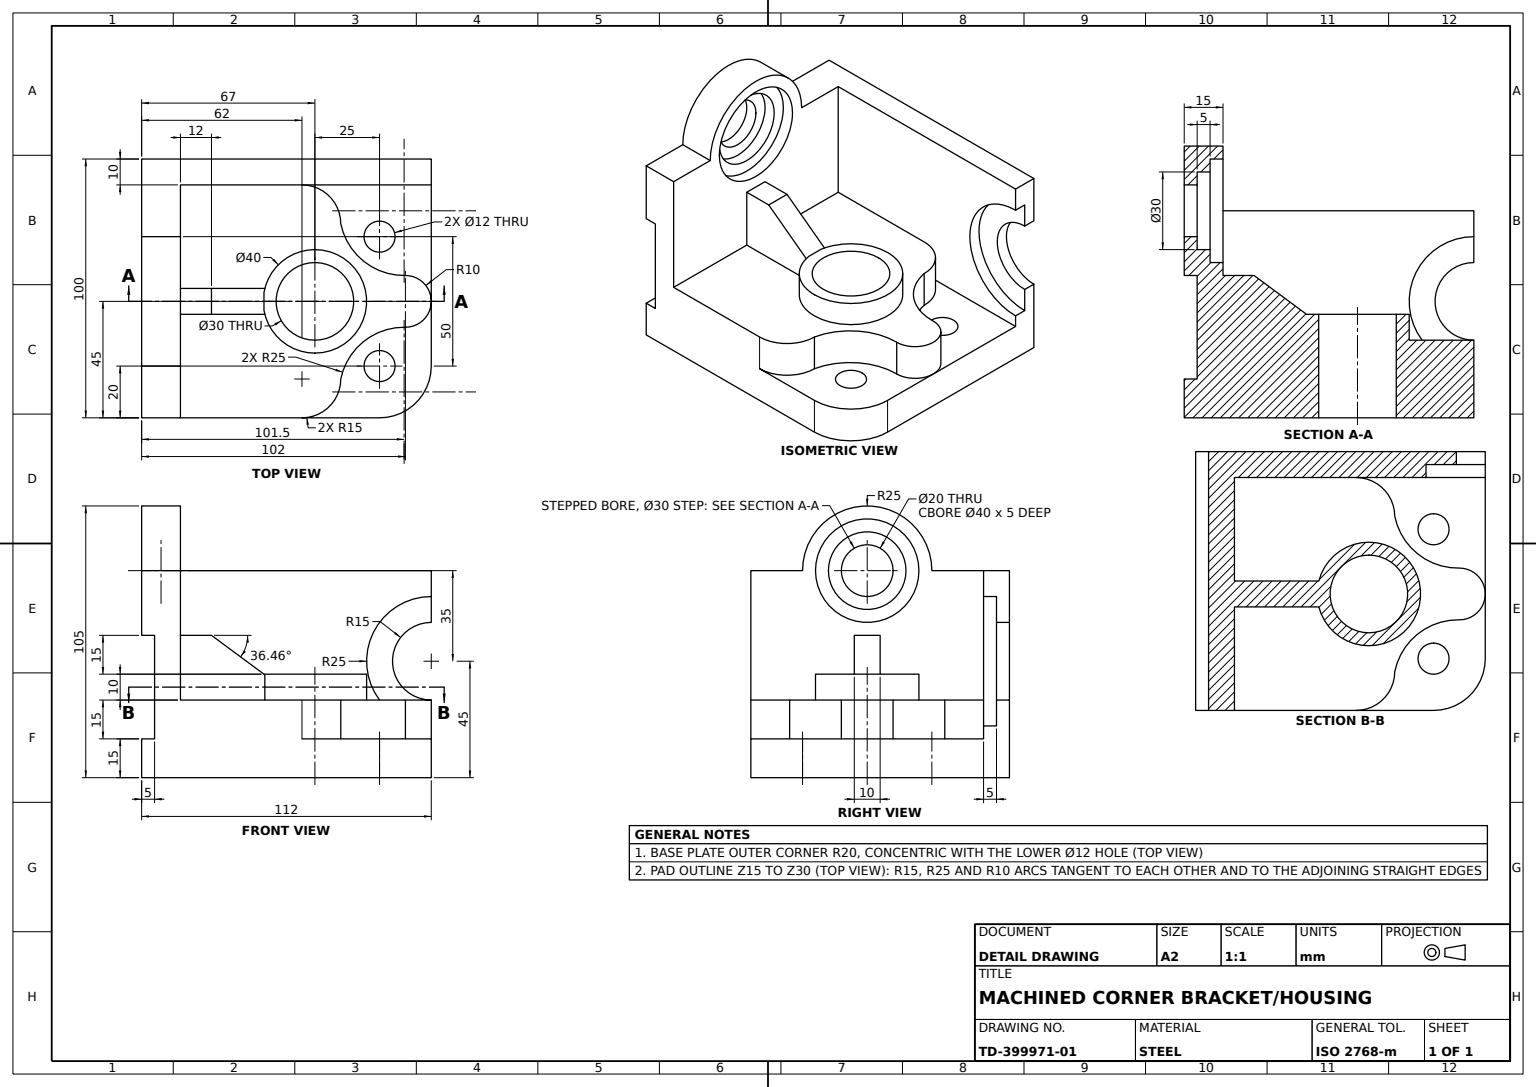
ISO-10303-21;
HEADER;
FILE_DESCRIPTION((''),'2;1');
FILE_NAME('','',(''),(''),'','','');
FILE_SCHEMA(('AUTOMOTIVE_DESIGN'));
ENDSEC;
DATA;
#1=APPLICATION_CONTEXT('');
#2=PRODUCT_CONTEXT('',#1,'mechanical');
#3=PRODUCT('','','',(#2));
#4=PRODUCT_DEFINITION_FORMATION('','',#3);
#5=PRODUCT_DEFINITION_CONTEXT('',#1,'design');
#6=PRODUCT_DEFINITION('','',#4,#5);
#7=PRODUCT_DEFINITION_SHAPE('','',#6);
#8=(LENGTH_UNIT()NAMED_UNIT(*)SI_UNIT(.MILLI.,.METRE.));
#9=(NAMED_UNIT(*)PLANE_ANGLE_UNIT()SI_UNIT($,.RADIAN.));
#10=(NAMED_UNIT(*)SI_UNIT($,.STERADIAN.)SOLID_ANGLE_UNIT());
#11=UNCERTAINTY_MEASURE_WITH_UNIT(LENGTH_MEASURE(1.E-05),#8,'distance_accuracy_value','');
#12=(GEOMETRIC_REPRESENTATION_CONTEXT(3)GLOBAL_UNCERTAINTY_ASSIGNED_CONTEXT((#11))GLOBAL_UNIT_ASSIGNED_CONTEXT((#8,#9,#10))REPRESENTATION_CONTEXT('',''));
#13=CARTESIAN_POINT('',(0.,40.,15.));
#14=VERTEX_POINT('',#13);
#15=CARTESIAN_POINT('',(0.,40.,-15.));
#16=VERTEX_POINT('',#15);
#17=CARTESIAN_POINT('',(0.,40.,0.));
#18=DIRECTION('',(0.,1.,0.));
#19=DIRECTION('',(0.,0.,1.));
#20=AXIS2_PLACEMENT_3D('',#17,#18,#19);
#21=CIRCLE('',#20,15.);
#22=EDGE_CURVE('',#14,#16,#21,.T.);
#23=ORIENTED_EDGE('',*,*,#22,.T.);
#24=CARTESIAN_POINT('',(0.,0.,-15.));
#25=VERTEX_POINT('',#24);
#26=DIRECTION('',(0.,-1.,0.));
#27=VECTOR('',#26,1000.);
#28=LINE('',#15,#27);
#29=EDGE_CURVE('',#16,#25,#28,.T.);
#30=ORIENTED_EDGE('',*,*,#29,.T.);
#31=CARTESIAN_POINT('',(0.,0.,15.));
#32=VERTEX_POINT('',#31);
#33=CARTESIAN_POINT('',(0.,0.,0.));
#34=AXIS2_PLACEMENT_3D('',#33,#18,#19);
#35=CIRCLE('',#34,15.);
#36=EDGE_CURVE('',#32,#25,#35,.T.);
#37=ORIENTED_EDGE('',*,*,#36,.F.);
#38=LINE('',#13,#27);
#39=EDGE_CURVE('',#14,#32,#38,.T.);
#40=ORIENTED_EDGE('',*,*,#39,.F.);
#41=EDGE_LOOP('',(#23,#30,#37,#40));
#42=FACE_OUTER_BOUND('',#41,.T.);
#43=DIRECTION('',(0.,0.,-1.));
#44=AXIS2_PLACEMENT_3D('',#17,#26,#43);
#45=CYLINDRICAL_SURFACE('',#44,15.);
#46=ADVANCED_FACE('',(#42),#45,.F.);
#47=CARTESIAN_POINT('',(-62.,80.,15.));
#48=VERTEX_POINT('',#47);
#49=CARTESIAN_POINT('',(-62.,80.,-15.));
#50=VERTEX_POINT('',#49);
#51=CARTESIAN_POINT('',(-62.,80.,0.));
#52=DIRECTION('',(1.,0.,0.));
#53=AXIS2_PLACEMENT_3D('',#51,#52,#43);
#54=CIRCLE('',#53,15.);
#55=EDGE_CURVE('',#48,#50,#54,.T.);
#56=ORIENTED_EDGE('',*,*,#55,.T.);
#57=EDGE_CURVE('',#50,#48,#54,.T.);
#58=ORIENTED_EDGE('',*,*,#57,.T.);
#59=EDGE_LOOP('',(#56,#58));
#60=FACE_OUTER_BOUND('',#59,.T.);
#61=CARTESIAN_POINT('',(-62.,80.,10.));
#62=VERTEX_POINT('',#61);
#63=CARTESIAN_POINT('',(-62.,80.,-10.));
#64=VERTEX_POINT('',#63);
#65=DIRECTION('',(-1.,0.,0.));
#66=AXIS2_PLACEMENT_3D('',#51,#65,#43);
#67=CIRCLE('',#66,10.);
#68=EDGE_CURVE('',#62,#64,#67,.T.);
#69=ORIENTED_EDGE('',*,*,#68,.T.);
#70=EDGE_CURVE('',#64,#62,#67,.T.);
#71=ORIENTED_EDGE('',*,*,#70,.T.);
#72=EDGE_LOOP('',(#69,#71));
#73=FACE_BOUND('',#72,.T.);
#74=PLANE('',#53);
#75=ADVANCED_FACE('',(#60,#73),#74,.T.);
#76=CARTESIAN_POINT('',(-52.,30.,5.));
#77=VERTEX_POINT('',#76);
#78=CARTESIAN_POINT('',(-19.364917,30.,5.));
#79=VERTEX_POINT('',#78);
#80=CARTESIAN_POINT('',(34.495934,30.,5.));
#81=VECTOR('',#52,1000.);
#82=LINE('',#80,#81);
#83=EDGE_CURVE('',#77,#79,#82,.T.);
#84=ORIENTED_EDGE('',*,*,#83,.T.);
#85=CARTESIAN_POINT('',(-19.364917,39.752402,5.));
#86=VERTEX_POINT('',#85);
#87=CARTESIAN_POINT('',(-19.364917,40.,5.));
#88=LINE('',#87,#27);
#89=EDGE_CURVE('',#86,#79,#88,.T.);
#90=ORIENTED_EDGE('',*,*,#89,.F.);
#91=CARTESIAN_POINT('',(-40.,55.,5.));
#92=VERTEX_POINT('',#91);
#93=DIRECTION('',(0.804258471,-0.594279658,0.));
#94=VECTOR('',#93,1000.);
#95=LINE('',#91,#94);
#96=EDGE_CURVE('',#92,#86,#95,.T.);
#97=ORIENTED_EDGE('',*,*,#96,.F.);
#98=CARTESIAN_POINT('',(-52.,55.,5.));
#99=VERTEX_POINT('',#98);
#100=CARTESIAN_POINT('',(-11.,55.,5.));
#101=LINE('',#100,#81);
#102=EDGE_CURVE('',#99,#92,#101,.T.);
#103=ORIENTED_EDGE('',*,*,#102,.F.);
#104=CARTESIAN_POINT('',(-52.,0.,5.));
#105=VECTOR('',#18,1000.);
#106=LINE('',#104,#105);
#107=EDGE_CURVE('',#77,#99,#106,.T.);
#108=ORIENTED_EDGE('',*,*,#107,.F.);
#109=EDGE_LOOP('',(#84,#90,#97,#103,#108));
#110=FACE_OUTER_BOUND('',#109,.T.);
#111=CARTESIAN_POINT('',(-11.,40.,5.));
#112=AXIS2_PLACEMENT_3D('',#111,#19,#52);
#113=PLANE('',#112);
#114=ADVANCED_FACE('',(#110),#113,.T.);
#115=CARTESIAN_POINT('',(-52.,80.,45.));
#116=VERTEX_POINT('',#115);
#117=CARTESIAN_POINT('',(-67.,80.,45.));
#118=VERTEX_POINT('',#117);
#119=CARTESIAN_POINT('',(0.,80.,45.));
#120=VECTOR('',#65,1000.);
#121=LINE('',#119,#120);
#122=EDGE_CURVE('',#116,#118,#121,.T.);
#123=ORIENTED_EDGE('',*,*,#122,.F.);
#124=CARTESIAN_POINT('',(-52.,80.,25.));
#125=VERTEX_POINT('',#124);
#126=CARTESIAN_POINT('',(-52.,80.,-45.));
#127=VECTOR('',#19,1000.);
#128=LINE('',#126,#127);
#129=EDGE_CURVE('',#125,#116,#128,.T.);
#130=ORIENTED_EDGE('',*,*,#129,.F.);
#131=CARTESIAN_POINT('',(-67.,80.,25.));
#132=VERTEX_POINT('',#131);
#133=LINE('',#131,#81);
#134=EDGE_CURVE('',#132,#125,#133,.T.);
#135=ORIENTED_EDGE('',*,*,#134,.F.);
#136=CARTESIAN_POINT('',(-67.,80.,-45.));
#137=LINE('',#136,#127);
#138=EDGE_CURVE('',#132,#118,#137,.T.);
#139=ORIENTED_EDGE('',*,*,#138,.T.);
#140=EDGE_LOOP('',(#123,#130,#135,#139));
#141=FACE_OUTER_BOUND('',#140,.T.);
#142=CARTESIAN_POINT('',(0.,80.,-45.));
#143=AXIS2_PLACEMENT_3D('',#142,#18,#19);
#144=PLANE('',#143);
#145=ADVANCED_FACE('',(#141),#144,.T.);
#146=CARTESIAN_POINT('',(-67.,0.,-55.));
#147=VERTEX_POINT('',#146);
#148=CARTESIAN_POINT('',(45.,0.,-55.));
#149=VERTEX_POINT('',#148);
#150=LINE('',#146,#81);
#151=EDGE_CURVE('',#147,#149,#150,.T.);
#152=ORIENTED_EDGE('',*,*,#151,.F.);
#153=CARTESIAN_POINT('',(-67.,15.,-55.));
#154=VERTEX_POINT('',#153);
#155=CARTESIAN_POINT('',(-67.,-112.445542,-55.));
#156=LINE('',#155,#105);
#157=EDGE_CURVE('',#147,#154,#156,.T.);
#158=ORIENTED_EDGE('',*,*,#157,.T.);
#159=CARTESIAN_POINT('',(-62.,15.,-55.));
#160=VERTEX_POINT('',#159);
#161=LINE('',#153,#120);
#162=EDGE_CURVE('',#160,#154,#161,.T.);
#163=ORIENTED_EDGE('',*,*,#162,.F.);
#164=CARTESIAN_POINT('',(-62.,55.,-55.));
#165=VERTEX_POINT('',#164);
#166=CARTESIAN_POINT('',(-62.,-112.445542,-55.));
#167=LINE('',#166,#27);
#168=EDGE_CURVE('',#165,#160,#167,.T.);
#169=ORIENTED_EDGE('',*,*,#168,.F.);
#170=CARTESIAN_POINT('',(-67.,55.,-55.));
#171=VERTEX_POINT('',#170);
#172=LINE('',#170,#81);
#173=EDGE_CURVE('',#171,#165,#172,.T.);
#174=ORIENTED_EDGE('',*,*,#173,.F.);
#175=CARTESIAN_POINT('',(-67.,80.,-55.));
#176=VERTEX_POINT('',#175);
#177=EDGE_CURVE('',#171,#176,#156,.T.);
#178=ORIENTED_EDGE('',*,*,#177,.T.);
#179=CARTESIAN_POINT('',(45.,80.,-55.));
#180=VERTEX_POINT('',#179);
#181=LINE('',#175,#120);
#182=EDGE_CURVE('',#180,#176,#181,.T.);
#183=ORIENTED_EDGE('',*,*,#182,.F.);
#184=CARTESIAN_POINT('',(45.,60.,-55.));
#185=VERTEX_POINT('',#184);
#186=CARTESIAN_POINT('',(45.,-112.445542,-55.));
#187=LINE('',#186,#105);
#188=EDGE_CURVE('',#185,#180,#187,.T.);
#189=ORIENTED_EDGE('',*,*,#188,.F.);
#190=CARTESIAN_POINT('',(45.,30.,-55.));
#191=VERTEX_POINT('',#190);
#192=CARTESIAN_POINT('',(45.,45.,-55.));
#193=AXIS2_PLACEMENT_3D('',#192,#19,#52);
#194=CIRCLE('',#193,15.);
#195=EDGE_CURVE('',#185,#191,#194,.T.);
#196=ORIENTED_EDGE('',*,*,#195,.T.);
#197=EDGE_CURVE('',#149,#191,#187,.T.);
#198=ORIENTED_EDGE('',*,*,#197,.F.);
#199=EDGE_LOOP('',(#152,#158,#163,#169,#174,#178,#183,#189,#196,#198));
#200=FACE_OUTER_BOUND('',#199,.T.);
#201=AXIS2_PLACEMENT_3D('',#155,#43,#65);
#202=PLANE('',#201);
#203=ADVANCED_FACE('',(#200),#202,.T.);
#204=CARTESIAN_POINT('',(-5.,30.,-45.));
#205=VERTEX_POINT('',#204);
#206=CARTESIAN_POINT('',(-5.,15.,-45.));
#207=VERTEX_POINT('',#206);
#208=LINE('',#204,#27);
#209=EDGE_CURVE('',#205,#207,#208,.T.);
#210=ORIENTED_EDGE('',*,*,#209,.F.);
#211=CARTESIAN_POINT('',(10.,30.,-30.));
#212=VERTEX_POINT('',#211);
#213=CARTESIAN_POINT('',(-5.,30.,-30.));
#214=AXIS2_PLACEMENT_3D('',#213,#18,#19);
#215=CIRCLE('',#214,15.);
#216=EDGE_CURVE('',#212,#205,#215,.T.);
#217=ORIENTED_EDGE('',*,*,#216,.F.);
#218=CARTESIAN_POINT('',(10.,15.,-30.));
#219=VERTEX_POINT('',#218);
#220=LINE('',#211,#27);
#221=EDGE_CURVE('',#212,#219,#220,.T.);
#222=ORIENTED_EDGE('',*,*,#221,.T.);
#223=CARTESIAN_POINT('',(-5.,15.,-30.));
#224=AXIS2_PLACEMENT_3D('',#223,#18,#19);
#225=CIRCLE('',#224,15.);
#226=EDGE_CURVE('',#219,#207,#225,.T.);
#227=ORIENTED_EDGE('',*,*,#226,.T.);
#228=EDGE_LOOP('',(#210,#217,#222,#227));
#229=FACE_OUTER_BOUND('',#228,.T.);
#230=AXIS2_PLACEMENT_3D('',#213,#26,#43);
#231=CYLINDRICAL_SURFACE('',#230,15.);
#232=ADVANCED_FACE('',(#229),#231,.T.);
#233=CARTESIAN_POINT('',(45.,15.,-45.));
#234=VERTEX_POINT('',#233);
#235=CARTESIAN_POINT('',(-45.,15.,-45.));
#236=LINE('',#235,#120);
#237=EDGE_CURVE('',#234,#207,#236,.T.);
#238=ORIENTED_EDGE('',*,*,#237,.T.);
#239=ORIENTED_EDGE('',*,*,#226,.F.);
#240=CARTESIAN_POINT('',(35.,15.,-10.));
#241=VERTEX_POINT('',#240);
#242=CARTESIAN_POINT('',(34.495934,15.,-34.994918));
#243=AXIS2_PLACEMENT_3D('',#242,#26,#19);
#244=CIRCLE('',#243,25.);
#245=EDGE_CURVE('',#241,#219,#244,.T.);
#246=ORIENTED_EDGE('',*,*,#245,.F.);
#247=CARTESIAN_POINT('',(45.,15.,0.));
#248=VERTEX_POINT('',#247);
#249=CARTESIAN_POINT('',(35.,15.,0.));
#250=AXIS2_PLACEMENT_3D('',#249,#18,#19);
#251=CIRCLE('',#250,10.);
#252=EDGE_CURVE('',#248,#241,#251,.T.);
#253=ORIENTED_EDGE('',*,*,#252,.F.);
#254=VECTOR('',#43,1000.);
#255=LINE('',#233,#254);
#256=EDGE_CURVE('',#248,#234,#255,.T.);
#257=ORIENTED_EDGE('',*,*,#256,.T.);
#258=EDGE_LOOP('',(#238,#239,#246,#253,#257));
#259=FACE_OUTER_BOUND('',#258,.T.);
#260=CARTESIAN_POINT('',(25.,15.,-31.));
#261=VERTEX_POINT('',#260);
#262=CARTESIAN_POINT('',(25.,15.,-19.));
#263=VERTEX_POINT('',#262);
#264=CARTESIAN_POINT('',(25.,15.,-25.));
#265=AXIS2_PLACEMENT_3D('',#264,#18,#19);
#266=CIRCLE('',#265,6.);
#267=EDGE_CURVE('',#261,#263,#266,.T.);
#268=ORIENTED_EDGE('',*,*,#267,.F.);
#269=EDGE_CURVE('',#263,#261,#266,.T.);
#270=ORIENTED_EDGE('',*,*,#269,.F.);
#271=EDGE_LOOP('',(#268,#270));
#272=FACE_BOUND('',#271,.T.);
#273=CARTESIAN_POINT('',(25.,15.,25.));
#274=AXIS2_PLACEMENT_3D('',#273,#18,#19);
#275=PLANE('',#274);
#276=ADVANCED_FACE('',(#259,#272),#275,.T.);
#277=CARTESIAN_POINT('',(45.,60.,-50.));
#278=VERTEX_POINT('',#277);
#279=CARTESIAN_POINT('',(45.,70.,-50.));
#280=VERTEX_POINT('',#279);
#281=CARTESIAN_POINT('',(45.,15.,-50.));
#282=LINE('',#281,#105);
#283=EDGE_CURVE('',#278,#280,#282,.T.);
#284=ORIENTED_EDGE('',*,*,#283,.T.);
#285=CARTESIAN_POINT('',(45.,20.,-50.));
#286=VERTEX_POINT('',#285);
#287=CARTESIAN_POINT('',(45.,45.,-50.));
#288=AXIS2_PLACEMENT_3D('',#287,#19,#52);
#289=CIRCLE('',#288,25.);
#290=EDGE_CURVE('',#280,#286,#289,.T.);
#291=ORIENTED_EDGE('',*,*,#290,.T.);
#292=CARTESIAN_POINT('',(45.,30.,-50.));
#293=VERTEX_POINT('',#292);
#294=EDGE_CURVE('',#286,#293,#282,.T.);
#295=ORIENTED_EDGE('',*,*,#294,.T.);
#296=CIRCLE('',#288,15.);
#297=EDGE_CURVE('',#278,#293,#296,.T.);
#298=ORIENTED_EDGE('',*,*,#297,.F.);
#299=EDGE_LOOP('',(#284,#291,#295,#298));
#300=FACE_OUTER_BOUND('',#299,.T.);
#301=PLANE('',#288);
#302=ADVANCED_FACE('',(#300),#301,.T.);
#303=CARTESIAN_POINT('',(-52.,30.,45.));
#304=VERTEX_POINT('',#303);
#305=CARTESIAN_POINT('',(-52.,0.,45.));
#306=LINE('',#305,#27);
#307=EDGE_CURVE('',#116,#304,#306,.T.);
#308=ORIENTED_EDGE('',*,*,#307,.T.);
#309=CARTESIAN_POINT('',(-52.,30.,-45.));
#310=LINE('',#309,#127);
#311=EDGE_CURVE('',#77,#304,#310,.T.);
#312=ORIENTED_EDGE('',*,*,#311,.F.);
#313=ORIENTED_EDGE('',*,*,#107,.T.);
#314=CARTESIAN_POINT('',(-52.,55.,-5.));
#315=VERTEX_POINT('',#314);
#316=CARTESIAN_POINT('',(-52.,55.,-45.));
#317=LINE('',#316,#254);
#318=EDGE_CURVE('',#99,#315,#317,.T.);
#319=ORIENTED_EDGE('',*,*,#318,.T.);
#320=CARTESIAN_POINT('',(-52.,30.,-5.));
#321=VERTEX_POINT('',#320);
#322=CARTESIAN_POINT('',(-52.,0.,-5.));
#323=LINE('',#322,#105);
#324=EDGE_CURVE('',#321,#315,#323,.T.);
#325=ORIENTED_EDGE('',*,*,#324,.F.);
#326=VERTEX_POINT('',#309);
#327=EDGE_CURVE('',#326,#321,#310,.T.);
#328=ORIENTED_EDGE('',*,*,#327,.F.);
#329=VERTEX_POINT('',#126);
#330=CARTESIAN_POINT('',(-52.,0.,-45.));
#331=LINE('',#330,#27);
#332=EDGE_CURVE('',#329,#326,#331,.T.);
#333=ORIENTED_EDGE('',*,*,#332,.F.);
#334=CARTESIAN_POINT('',(-52.,80.,-25.));
#335=VERTEX_POINT('',#334);
#336=EDGE_CURVE('',#329,#335,#128,.T.);
#337=ORIENTED_EDGE('',*,*,#336,.T.);
#338=CARTESIAN_POINT('',(-52.,80.,0.));
#339=AXIS2_PLACEMENT_3D('',#338,#52,#43);
#340=CIRCLE('',#339,25.);
#341=EDGE_CURVE('',#335,#125,#340,.T.);
#342=ORIENTED_EDGE('',*,*,#341,.T.);
#343=ORIENTED_EDGE('',*,*,#129,.T.);
#344=EDGE_LOOP('',(#308,#312,#313,#319,#325,#328,#333,#337,#342,#343));
#345=FACE_OUTER_BOUND('',#344,.T.);
#346=CARTESIAN_POINT('',(-52.,80.,20.));
#347=VERTEX_POINT('',#346);
#348=CARTESIAN_POINT('',(-52.,80.,-20.));
#349=VERTEX_POINT('',#348);
#350=CIRCLE('',#339,20.);
#351=EDGE_CURVE('',#347,#349,#350,.T.);
#352=ORIENTED_EDGE('',*,*,#351,.F.);
#353=EDGE_CURVE('',#349,#347,#350,.T.);
#354=ORIENTED_EDGE('',*,*,#353,.F.);
#355=EDGE_LOOP('',(#352,#354));
#356=FACE_BOUND('',#355,.T.);
#357=AXIS2_PLACEMENT_3D('',#330,#65,#19);
#358=PLANE('',#357);
#359=ADVANCED_FACE('',(#345,#356),#358,.F.);
#360=CARTESIAN_POINT('',(25.,15.,19.));
#361=VERTEX_POINT('',#360);
#362=CARTESIAN_POINT('',(25.,15.,31.));
#363=VERTEX_POINT('',#362);
#364=CIRCLE('',#274,6.);
#365=EDGE_CURVE('',#361,#363,#364,.T.);
#366=ORIENTED_EDGE('',*,*,#365,.F.);
#367=EDGE_CURVE('',#363,#361,#364,.T.);
#368=ORIENTED_EDGE('',*,*,#367,.F.);
#369=EDGE_LOOP('',(#366,#368));
#370=FACE_BOUND('',#369,.T.);
#371=CARTESIAN_POINT('',(45.,15.,25.));
#372=VERTEX_POINT('',#371);
#373=EDGE_CURVE('',#372,#248,#255,.T.);
#374=ORIENTED_EDGE('',*,*,#373,.T.);
#375=CARTESIAN_POINT('',(35.,15.,10.));
#376=VERTEX_POINT('',#375);
#377=EDGE_CURVE('',#376,#248,#251,.T.);
#378=ORIENTED_EDGE('',*,*,#377,.F.);
#379=CARTESIAN_POINT('',(34.495934,15.,9.994918));
#380=VERTEX_POINT('',#379);
#381=CARTESIAN_POINT('',(34.495934,15.,34.994918));
#382=AXIS2_PLACEMENT_3D('',#381,#26,#43);
#383=CIRCLE('',#382,25.);
#384=EDGE_CURVE('',#380,#376,#383,.T.);
#385=ORIENTED_EDGE('',*,*,#384,.F.);
#386=CARTESIAN_POINT('',(10.,15.,30.));
#387=VERTEX_POINT('',#386);
#388=EDGE_CURVE('',#387,#380,#383,.T.);
#389=ORIENTED_EDGE('',*,*,#388,.F.);
#390=CARTESIAN_POINT('',(-5.,15.,45.));
#391=VERTEX_POINT('',#390);
#392=CARTESIAN_POINT('',(-5.,15.,30.));
#393=AXIS2_PLACEMENT_3D('',#392,#18,#19);
#394=CIRCLE('',#393,15.);
#395=EDGE_CURVE('',#391,#387,#394,.T.);
#396=ORIENTED_EDGE('',*,*,#395,.F.);
#397=CARTESIAN_POINT('',(25.,15.,45.));
#398=VERTEX_POINT('',#397);
#399=CARTESIAN_POINT('',(-45.,15.,45.));
#400=LINE('',#399,#81);
#401=EDGE_CURVE('',#391,#398,#400,.T.);
#402=ORIENTED_EDGE('',*,*,#401,.T.);
#403=CIRCLE('',#274,20.);
#404=EDGE_CURVE('',#398,#372,#403,.T.);
#405=ORIENTED_EDGE('',*,*,#404,.T.);
#406=EDGE_LOOP('',(#374,#378,#385,#389,#396,#402,#405));
#407=FACE_OUTER_BOUND('',#406,.T.);
#408=ADVANCED_FACE('',(#370,#407),#275,.T.);
#409=CARTESIAN_POINT('',(25.,0.,31.));
#410=VERTEX_POINT('',#409);
#411=CARTESIAN_POINT('',(25.,0.,19.));
#412=VERTEX_POINT('',#411);
#413=CARTESIAN_POINT('',(25.,0.,25.));
#414=AXIS2_PLACEMENT_3D('',#413,#18,#19);
#415=CIRCLE('',#414,6.);
#416=EDGE_CURVE('',#410,#412,#415,.T.);
#417=ORIENTED_EDGE('',*,*,#416,.F.);
#418=LINE('',#362,#27);
#419=EDGE_CURVE('',#363,#410,#418,.T.);
#420=ORIENTED_EDGE('',*,*,#419,.F.);
#421=ORIENTED_EDGE('',*,*,#367,.T.);
#422=LINE('',#360,#27);
#423=EDGE_CURVE('',#361,#412,#422,.T.);
#424=ORIENTED_EDGE('',*,*,#423,.T.);
#425=EDGE_LOOP('',(#417,#420,#421,#424));
#426=FACE_OUTER_BOUND('',#425,.T.);
#427=AXIS2_PLACEMENT_3D('',#273,#26,#43);
#428=CYLINDRICAL_SURFACE('',#427,6.);
#429=ADVANCED_FACE('',(#426),#428,.F.);
#430=CARTESIAN_POINT('',(45.,20.,-45.));
#431=VERTEX_POINT('',#430);
#432=LINE('',#285,#127);
#433=EDGE_CURVE('',#286,#431,#432,.T.);
#434=ORIENTED_EDGE('',*,*,#433,.T.);
#435=CARTESIAN_POINT('',(45.,-112.445542,-45.));
#436=LINE('',#435,#105);
#437=EDGE_CURVE('',#234,#431,#436,.T.);
#438=ORIENTED_EDGE('',*,*,#437,.F.);
#439=ORIENTED_EDGE('',*,*,#256,.F.);
#440=ORIENTED_EDGE('',*,*,#373,.F.);
#441=CARTESIAN_POINT('',(45.,0.,25.));
#442=VERTEX_POINT('',#441);
#443=LINE('',#371,#27);
#444=EDGE_CURVE('',#372,#442,#443,.T.);
#445=ORIENTED_EDGE('',*,*,#444,.T.);
#446=CARTESIAN_POINT('',(45.,0.,-45.));
#447=LINE('',#446,#254);
#448=EDGE_CURVE('',#442,#149,#447,.T.);
#449=ORIENTED_EDGE('',*,*,#448,.T.);
#450=ORIENTED_EDGE('',*,*,#197,.T.);
#451=LINE('',#190,#127);
#452=EDGE_CURVE('',#191,#293,#451,.T.);
#453=ORIENTED_EDGE('',*,*,#452,.T.);
#454=ORIENTED_EDGE('',*,*,#294,.F.);
#455=EDGE_LOOP('',(#434,#438,#439,#440,#445,#449,#450,#453,#454));
#456=FACE_OUTER_BOUND('',#455,.T.);
#457=AXIS2_PLACEMENT_3D('',#233,#65,#19);
#458=PLANE('',#457);
#459=ADVANCED_FACE('',(#456),#458,.F.);
#460=CARTESIAN_POINT('',(-62.,55.,45.));
#461=VERTEX_POINT('',#460);
#462=CARTESIAN_POINT('',(-62.,55.,-45.));
#463=LINE('',#462,#127);
#464=EDGE_CURVE('',#165,#461,#463,.T.);
#465=ORIENTED_EDGE('',*,*,#464,.F.);
#466=ORIENTED_EDGE('',*,*,#168,.T.);
#467=CARTESIAN_POINT('',(-62.,15.,45.));
#468=VERTEX_POINT('',#467);
#469=CARTESIAN_POINT('',(-62.,15.,-45.));
#470=LINE('',#469,#127);
#471=EDGE_CURVE('',#160,#468,#470,.T.);
#472=ORIENTED_EDGE('',*,*,#471,.T.);
#473=CARTESIAN_POINT('',(-62.,0.,45.));
#474=LINE('',#473,#27);
#475=EDGE_CURVE('',#461,#468,#474,.T.);
#476=ORIENTED_EDGE('',*,*,#475,.F.);
#477=EDGE_LOOP('',(#465,#466,#472,#476));
#478=FACE_OUTER_BOUND('',#477,.T.);
#479=CARTESIAN_POINT('',(-62.,0.,-45.));
#480=AXIS2_PLACEMENT_3D('',#479,#65,#19);
#481=PLANE('',#480);
#482=ADVANCED_FACE('',(#478),#481,.T.);
#483=ORIENTED_EDGE('',*,*,#452,.F.);
#484=ORIENTED_EDGE('',*,*,#195,.F.);
#485=LINE('',#184,#254);
#486=EDGE_CURVE('',#278,#185,#485,.T.);
#487=ORIENTED_EDGE('',*,*,#486,.F.);
#488=ORIENTED_EDGE('',*,*,#297,.T.);
#489=EDGE_LOOP('',(#483,#484,#487,#488));
#490=FACE_OUTER_BOUND('',#489,.T.);
#491=CYLINDRICAL_SURFACE('',#193,15.);
#492=ADVANCED_FACE('',(#490),#491,.F.);
#493=CARTESIAN_POINT('',(-67.,80.,-25.));
#494=VERTEX_POINT('',#493);
#495=CARTESIAN_POINT('',(-67.,80.,0.));
#496=AXIS2_PLACEMENT_3D('',#495,#52,#43);
#497=CIRCLE('',#496,25.);
#498=EDGE_CURVE('',#494,#132,#497,.T.);
#499=ORIENTED_EDGE('',*,*,#498,.T.);
#500=ORIENTED_EDGE('',*,*,#134,.T.);
#501=ORIENTED_EDGE('',*,*,#341,.F.);
#502=LINE('',#493,#81);
#503=EDGE_CURVE('',#494,#335,#502,.T.);
#504=ORIENTED_EDGE('',*,*,#503,.F.);
#505=EDGE_LOOP('',(#499,#500,#501,#504));
#506=FACE_OUTER_BOUND('',#505,.T.);
#507=CYLINDRICAL_SURFACE('',#496,25.);
#508=ADVANCED_FACE('',(#506),#507,.T.);
#509=CARTESIAN_POINT('',(-40.,55.,-5.));
#510=VERTEX_POINT('',#509);
#511=CARTESIAN_POINT('',(-11.,55.,-5.));
#512=LINE('',#511,#81);
#513=EDGE_CURVE('',#315,#510,#512,.T.);
#514=ORIENTED_EDGE('',*,*,#513,.T.);
#515=CARTESIAN_POINT('',(-19.364917,39.752402,-5.));
#516=VERTEX_POINT('',#515);
#517=LINE('',#509,#94);
#518=EDGE_CURVE('',#510,#516,#517,.T.);
#519=ORIENTED_EDGE('',*,*,#518,.T.);
#520=CARTESIAN_POINT('',(-19.364917,30.,-5.));
#521=VERTEX_POINT('',#520);
#522=CARTESIAN_POINT('',(-19.364917,40.,-5.));
#523=LINE('',#522,#27);
#524=EDGE_CURVE('',#516,#521,#523,.T.);
#525=ORIENTED_EDGE('',*,*,#524,.T.);
#526=CARTESIAN_POINT('',(34.495934,30.,-5.));
#527=LINE('',#526,#81);
#528=EDGE_CURVE('',#321,#521,#527,.T.);
#529=ORIENTED_EDGE('',*,*,#528,.F.);
#530=ORIENTED_EDGE('',*,*,#324,.T.);
#531=EDGE_LOOP('',(#514,#519,#525,#529,#530));
#532=FACE_OUTER_BOUND('',#531,.T.);
#533=CARTESIAN_POINT('',(-11.,40.,-5.));
#534=AXIS2_PLACEMENT_3D('',#533,#19,#52);
#535=PLANE('',#534);
#536=ADVANCED_FACE('',(#532),#535,.F.);
#537=CARTESIAN_POINT('',(-67.,55.,45.));
#538=VERTEX_POINT('',#537);
#539=CARTESIAN_POINT('',(-67.,55.,-45.));
#540=LINE('',#539,#127);
#541=EDGE_CURVE('',#171,#538,#540,.T.);
#542=ORIENTED_EDGE('',*,*,#541,.F.);
#543=ORIENTED_EDGE('',*,*,#173,.T.);
#544=ORIENTED_EDGE('',*,*,#464,.T.);
#545=CARTESIAN_POINT('',(0.,55.,45.));
#546=LINE('',#545,#81);
#547=EDGE_CURVE('',#538,#461,#546,.T.);
#548=ORIENTED_EDGE('',*,*,#547,.F.);
#549=EDGE_LOOP('',(#542,#543,#544,#548));
#550=FACE_OUTER_BOUND('',#549,.T.);
#551=CARTESIAN_POINT('',(0.,55.,-45.));
#552=AXIS2_PLACEMENT_3D('',#551,#26,#43);
#553=PLANE('',#552);
#554=ADVANCED_FACE('',(#550),#553,.T.);
#555=CARTESIAN_POINT('',(-57.,80.,-15.));
#556=VERTEX_POINT('',#555);
#557=LINE('',#49,#81);
#558=EDGE_CURVE('',#50,#556,#557,.T.);
#559=ORIENTED_EDGE('',*,*,#558,.T.);
#560=CARTESIAN_POINT('',(-57.,80.,15.));
#561=VERTEX_POINT('',#560);
#562=CARTESIAN_POINT('',(-57.,80.,0.));
#563=AXIS2_PLACEMENT_3D('',#562,#52,#43);
#564=CIRCLE('',#563,15.);
#565=EDGE_CURVE('',#556,#561,#564,.T.);
#566=ORIENTED_EDGE('',*,*,#565,.T.);
#567=LINE('',#47,#81);
#568=EDGE_CURVE('',#48,#561,#567,.T.);
#569=ORIENTED_EDGE('',*,*,#568,.F.);
#570=ORIENTED_EDGE('',*,*,#57,.F.);
#571=EDGE_LOOP('',(#559,#566,#569,#570));
#572=FACE_OUTER_BOUND('',#571,.T.);
#573=CYLINDRICAL_SURFACE('',#53,15.);
#574=ADVANCED_FACE('',(#572),#573,.F.);
#575=ORIENTED_EDGE('',*,*,#252,.T.);
#576=CARTESIAN_POINT('',(35.,30.,-10.));
#577=VERTEX_POINT('',#576);
#578=LINE('',#576,#27);
#579=EDGE_CURVE('',#577,#241,#578,.T.);
#580=ORIENTED_EDGE('',*,*,#579,.F.);
#581=CARTESIAN_POINT('',(35.,30.,10.));
#582=VERTEX_POINT('',#581);
#583=CARTESIAN_POINT('',(35.,30.,0.));
#584=AXIS2_PLACEMENT_3D('',#583,#18,#19);
#585=CIRCLE('',#584,10.);
#586=EDGE_CURVE('',#582,#577,#585,.T.);
#587=ORIENTED_EDGE('',*,*,#586,.F.);
#588=LINE('',#581,#27);
#589=EDGE_CURVE('',#582,#376,#588,.T.);
#590=ORIENTED_EDGE('',*,*,#589,.T.);
#591=ORIENTED_EDGE('',*,*,#377,.T.);
#592=EDGE_LOOP('',(#575,#580,#587,#590,#591));
#593=FACE_OUTER_BOUND('',#592,.T.);
#594=AXIS2_PLACEMENT_3D('',#583,#26,#43);
#595=CYLINDRICAL_SURFACE('',#594,10.);
#596=ADVANCED_FACE('',(#593),#595,.T.);
#597=EDGE_CURVE('',#16,#14,#21,.T.);
#598=ORIENTED_EDGE('',*,*,#597,.F.);
#599=ORIENTED_EDGE('',*,*,#22,.F.);
#600=EDGE_LOOP('',(#598,#599));
#601=FACE_BOUND('',#600,.T.);
#602=CARTESIAN_POINT('',(-19.7,40.,3.451087));
#603=VERTEX_POINT('',#602);
#604=CARTESIAN_POINT('',(-19.7,40.,-3.451087));
#605=VERTEX_POINT('',#604);
#606=CARTESIAN_POINT('',(-19.7,40.,0.));
#607=LINE('',#606,#254);
#608=EDGE_CURVE('',#603,#605,#607,.T.);
#609=ORIENTED_EDGE('',*,*,#608,.F.);
#610=CARTESIAN_POINT('',(0.,40.,20.));
#611=VERTEX_POINT('',#610);
#612=CIRCLE('',#20,20.);
#613=EDGE_CURVE('',#603,#611,#612,.T.);
#614=ORIENTED_EDGE('',*,*,#613,.T.);
#615=CARTESIAN_POINT('',(0.,40.,-20.));
#616=VERTEX_POINT('',#615);
#617=EDGE_CURVE('',#611,#616,#612,.T.);
#618=ORIENTED_EDGE('',*,*,#617,.T.);
#619=EDGE_CURVE('',#616,#605,#612,.T.);
#620=ORIENTED_EDGE('',*,*,#619,.T.);
#621=EDGE_LOOP('',(#609,#614,#618,#620));
#622=FACE_OUTER_BOUND('',#621,.T.);
#623=PLANE('',#20);
#624=ADVANCED_FACE('',(#601,#622),#623,.T.);
#625=ORIENTED_EDGE('',*,*,#365,.T.);
#626=ORIENTED_EDGE('',*,*,#419,.T.);
#627=EDGE_CURVE('',#412,#410,#415,.T.);
#628=ORIENTED_EDGE('',*,*,#627,.F.);
#629=ORIENTED_EDGE('',*,*,#423,.F.);
#630=EDGE_LOOP('',(#625,#626,#628,#629));
#631=FACE_OUTER_BOUND('',#630,.T.);
#632=ADVANCED_FACE('',(#631),#428,.F.);
#633=CARTESIAN_POINT('',(-57.,80.,-20.));
#634=VERTEX_POINT('',#633);
#635=LINE('',#633,#81);
#636=EDGE_CURVE('',#634,#349,#635,.T.);
#637=ORIENTED_EDGE('',*,*,#636,.T.);
#638=ORIENTED_EDGE('',*,*,#353,.T.);
#639=CARTESIAN_POINT('',(-57.,80.,20.));
#640=VERTEX_POINT('',#639);
#641=LINE('',#639,#81);
#642=EDGE_CURVE('',#640,#347,#641,.T.);
#643=ORIENTED_EDGE('',*,*,#642,.F.);
#644=CIRCLE('',#563,20.);
#645=EDGE_CURVE('',#634,#640,#644,.T.);
#646=ORIENTED_EDGE('',*,*,#645,.F.);
#647=EDGE_LOOP('',(#637,#638,#643,#646));
#648=FACE_OUTER_BOUND('',#647,.T.);
#649=CYLINDRICAL_SURFACE('',#563,20.);
#650=ADVANCED_FACE('',(#648),#649,.F.);
#651=CARTESIAN_POINT('',(-67.,80.,-10.));
#652=VERTEX_POINT('',#651);
#653=CARTESIAN_POINT('',(-67.,80.,10.));
#654=VERTEX_POINT('',#653);
#655=CIRCLE('',#496,10.);
#656=EDGE_CURVE('',#652,#654,#655,.T.);
#657=ORIENTED_EDGE('',*,*,#656,.F.);
#658=LINE('',#651,#81);
#659=EDGE_CURVE('',#652,#64,#658,.T.);
#660=ORIENTED_EDGE('',*,*,#659,.T.);
#661=ORIENTED_EDGE('',*,*,#68,.F.);
#662=LINE('',#653,#81);
#663=EDGE_CURVE('',#654,#62,#662,.T.);
#664=ORIENTED_EDGE('',*,*,#663,.F.);
#665=EDGE_LOOP('',(#657,#660,#661,#664));
#666=FACE_OUTER_BOUND('',#665,.T.);
#667=CYLINDRICAL_SURFACE('',#496,10.);
#668=ADVANCED_FACE('',(#666),#667,.F.);
#669=CARTESIAN_POINT('',(-67.,15.,45.));
#670=VERTEX_POINT('',#669);
#671=CARTESIAN_POINT('',(0.,15.,45.));
#672=LINE('',#671,#81);
#673=EDGE_CURVE('',#670,#468,#672,.T.);
#674=ORIENTED_EDGE('',*,*,#673,.T.);
#675=ORIENTED_EDGE('',*,*,#471,.F.);
#676=ORIENTED_EDGE('',*,*,#162,.T.);
#677=CARTESIAN_POINT('',(-67.,15.,-45.));
#678=LINE('',#677,#127);
#679=EDGE_CURVE('',#154,#670,#678,.T.);
#680=ORIENTED_EDGE('',*,*,#679,.T.);
#681=EDGE_LOOP('',(#674,#675,#676,#680));
#682=FACE_OUTER_BOUND('',#681,.T.);
#683=CARTESIAN_POINT('',(0.,15.,-45.));
#684=AXIS2_PLACEMENT_3D('',#683,#26,#43);
#685=PLANE('',#684);
#686=ADVANCED_FACE('',(#682),#685,.F.);
#687=LINE('',#204,#120);
#688=EDGE_CURVE('',#205,#326,#687,.T.);
#689=ORIENTED_EDGE('',*,*,#688,.T.);
#690=ORIENTED_EDGE('',*,*,#327,.T.);
#691=ORIENTED_EDGE('',*,*,#528,.T.);
#692=CARTESIAN_POINT('',(0.,30.,-20.));
#693=VERTEX_POINT('',#692);
#694=CARTESIAN_POINT('',(0.,30.,0.));
#695=AXIS2_PLACEMENT_3D('',#694,#18,#19);
#696=CIRCLE('',#695,20.);
#697=EDGE_CURVE('',#693,#521,#696,.T.);
#698=ORIENTED_EDGE('',*,*,#697,.F.);
#699=CARTESIAN_POINT('',(0.,30.,20.));
#700=VERTEX_POINT('',#699);
#701=EDGE_CURVE('',#700,#693,#696,.T.);
#702=ORIENTED_EDGE('',*,*,#701,.F.);
#703=EDGE_CURVE('',#79,#700,#696,.T.);
#704=ORIENTED_EDGE('',*,*,#703,.F.);
#705=ORIENTED_EDGE('',*,*,#83,.F.);
#706=ORIENTED_EDGE('',*,*,#311,.T.);
#707=CARTESIAN_POINT('',(-5.,30.,45.));
#708=VERTEX_POINT('',#707);
#709=CARTESIAN_POINT('',(-45.,30.,45.));
#710=LINE('',#709,#81);
#711=EDGE_CURVE('',#304,#708,#710,.T.);
#712=ORIENTED_EDGE('',*,*,#711,.T.);
#713=CARTESIAN_POINT('',(10.,30.,30.));
#714=VERTEX_POINT('',#713);
#715=CARTESIAN_POINT('',(-5.,30.,30.));
#716=AXIS2_PLACEMENT_3D('',#715,#18,#19);
#717=CIRCLE('',#716,15.);
#718=EDGE_CURVE('',#708,#714,#717,.T.);
#719=ORIENTED_EDGE('',*,*,#718,.T.);
#720=CARTESIAN_POINT('',(34.495934,30.,9.994918));
#721=VERTEX_POINT('',#720);
#722=CARTESIAN_POINT('',(34.495934,30.,34.994918));
#723=AXIS2_PLACEMENT_3D('',#722,#26,#43);
#724=CIRCLE('',#723,25.);
#725=EDGE_CURVE('',#714,#721,#724,.T.);
#726=ORIENTED_EDGE('',*,*,#725,.T.);
#727=EDGE_CURVE('',#721,#582,#724,.T.);
#728=ORIENTED_EDGE('',*,*,#727,.T.);
#729=ORIENTED_EDGE('',*,*,#586,.T.);
#730=CARTESIAN_POINT('',(34.495934,30.,-34.994918));
#731=AXIS2_PLACEMENT_3D('',#730,#26,#19);
#732=CIRCLE('',#731,25.);
#733=EDGE_CURVE('',#577,#212,#732,.T.);
#734=ORIENTED_EDGE('',*,*,#733,.T.);
#735=ORIENTED_EDGE('',*,*,#216,.T.);
#736=EDGE_LOOP('',(#689,#690,#691,#698,#702,#704,#705,#706,#712,#719,#726,#728,#729,#734,#735));
#737=FACE_OUTER_BOUND('',#736,.T.);
#738=AXIS2_PLACEMENT_3D('',#730,#18,#19);
#739=PLANE('',#738);
#740=ADVANCED_FACE('',(#737),#739,.T.);
#741=ORIENTED_EDGE('',*,*,#642,.T.);
#742=ORIENTED_EDGE('',*,*,#351,.T.);
#743=ORIENTED_EDGE('',*,*,#636,.F.);
#744=EDGE_CURVE('',#640,#634,#644,.T.);
#745=ORIENTED_EDGE('',*,*,#744,.F.);
#746=EDGE_LOOP('',(#741,#742,#743,#745));
#747=FACE_OUTER_BOUND('',#746,.T.);
#748=ADVANCED_FACE('',(#747),#649,.F.);
#749=ORIENTED_EDGE('',*,*,#565,.F.);
#750=EDGE_CURVE('',#561,#556,#564,.T.);
#751=ORIENTED_EDGE('',*,*,#750,.F.);
#752=EDGE_LOOP('',(#749,#751));
#753=FACE_BOUND('',#752,.T.);
#754=ORIENTED_EDGE('',*,*,#645,.T.);
#755=ORIENTED_EDGE('',*,*,#744,.T.);
#756=EDGE_LOOP('',(#754,#755));
#757=FACE_OUTER_BOUND('',#756,.T.);
#758=PLANE('',#563);
#759=ADVANCED_FACE('',(#753,#757),#758,.T.);
#760=ORIENTED_EDGE('',*,*,#332,.T.);
#761=ORIENTED_EDGE('',*,*,#688,.F.);
#762=ORIENTED_EDGE('',*,*,#209,.T.);
#763=ORIENTED_EDGE('',*,*,#237,.F.);
#764=ORIENTED_EDGE('',*,*,#437,.T.);
#765=CARTESIAN_POINT('',(45.,70.,-45.));
#766=VERTEX_POINT('',#765);
#767=CARTESIAN_POINT('',(45.,45.,-45.));
#768=AXIS2_PLACEMENT_3D('',#767,#19,#52);
#769=CIRCLE('',#768,25.);
#770=EDGE_CURVE('',#766,#431,#769,.T.);
#771=ORIENTED_EDGE('',*,*,#770,.F.);
#772=CARTESIAN_POINT('',(45.,80.,-45.));
#773=VERTEX_POINT('',#772);
#774=EDGE_CURVE('',#766,#773,#436,.T.);
#775=ORIENTED_EDGE('',*,*,#774,.T.);
#776=LINE('',#136,#81);
#777=EDGE_CURVE('',#329,#773,#776,.T.);
#778=ORIENTED_EDGE('',*,*,#777,.F.);
#779=EDGE_LOOP('',(#760,#761,#762,#763,#764,#771,#775,#778));
#780=FACE_OUTER_BOUND('',#779,.T.);
#781=CARTESIAN_POINT('',(-67.,-112.445542,-45.));
#782=AXIS2_PLACEMENT_3D('',#781,#19,#52);
#783=PLANE('',#782);
#784=ADVANCED_FACE('',(#780),#783,.T.);
#785=ORIENTED_EDGE('',*,*,#558,.F.);
#786=ORIENTED_EDGE('',*,*,#55,.F.);
#787=ORIENTED_EDGE('',*,*,#568,.T.);
#788=ORIENTED_EDGE('',*,*,#750,.T.);
#789=EDGE_LOOP('',(#785,#786,#787,#788));
#790=FACE_OUTER_BOUND('',#789,.T.);
#791=ADVANCED_FACE('',(#790),#573,.F.);
#792=ORIENTED_EDGE('',*,*,#518,.F.);
#793=CARTESIAN_POINT('',(-40.,55.,0.));
#794=LINE('',#793,#127);
#795=EDGE_CURVE('',#510,#92,#794,.T.);
#796=ORIENTED_EDGE('',*,*,#795,.T.);
#797=ORIENTED_EDGE('',*,*,#96,.T.);
#798=CARTESIAN_POINT('',(-19.608801,39.932611,3.971683));
#799=CARTESIAN_POINT('',(-19.497048,39.850035,4.488258));
#800=(BOUNDED_CURVE()B_SPLINE_CURVE(3,(#602,#798,#799,#85),.UNSPECIFIED.,.F.,.F.)B_SPLINE_CURVE_WITH_KNOTS((4,4),(3.315014975,3.394272909),.UNSPECIFIED.)CURVE()GEOMETRIC_REPRESENTATION_ITEM()RATIONAL_B_SPLINE_CURVE((1.,0.999476583,0.999476583,1.))REPRESENTATION_ITEM(''));
#801=EDGE_CURVE('',#603,#86,#800,.T.);
#802=ORIENTED_EDGE('',*,*,#801,.F.);
#803=ORIENTED_EDGE('',*,*,#608,.T.);
#804=CARTESIAN_POINT('',(-19.497048,39.850035,-4.488258));
#805=CARTESIAN_POINT('',(-19.608801,39.932611,-3.971683));
#806=(BOUNDED_CURVE()B_SPLINE_CURVE(3,(#515,#804,#805,#604),.UNSPECIFIED.,.F.,.F.)B_SPLINE_CURVE_WITH_KNOTS((4,4),(2.888912398,2.968170332),.UNSPECIFIED.)CURVE()GEOMETRIC_REPRESENTATION_ITEM()RATIONAL_B_SPLINE_CURVE((1.,0.999476583,0.999476583,1.))REPRESENTATION_ITEM(''));
#807=EDGE_CURVE('',#516,#605,#806,.T.);
#808=ORIENTED_EDGE('',*,*,#807,.F.);
#809=EDGE_LOOP('',(#792,#796,#797,#802,#803,#808));
#810=FACE_OUTER_BOUND('',#809,.T.);
#811=DIRECTION('',(-0.594279658,-0.804258471,0.));
#812=AXIS2_PLACEMENT_3D('',#793,#811,#93);
#813=PLANE('',#812);
#814=ADVANCED_FACE('',(#810),#813,.F.);
#815=ORIENTED_EDGE('',*,*,#416,.T.);
#816=ORIENTED_EDGE('',*,*,#627,.T.);
#817=EDGE_LOOP('',(#815,#816));
#818=FACE_BOUND('',#817,.T.);
#819=CARTESIAN_POINT('',(25.,0.,-19.));
#820=VERTEX_POINT('',#819);
#821=CARTESIAN_POINT('',(25.,0.,-31.));
#822=VERTEX_POINT('',#821);
#823=CARTESIAN_POINT('',(25.,0.,-25.));
#824=AXIS2_PLACEMENT_3D('',#823,#18,#19);
#825=CIRCLE('',#824,6.);
#826=EDGE_CURVE('',#820,#822,#825,.T.);
#827=ORIENTED_EDGE('',*,*,#826,.T.);
#828=EDGE_CURVE('',#822,#820,#825,.T.);
#829=ORIENTED_EDGE('',*,*,#828,.T.);
#830=EDGE_LOOP('',(#827,#829));
#831=FACE_BOUND('',#830,.T.);
#832=EDGE_CURVE('',#25,#32,#35,.T.);
#833=ORIENTED_EDGE('',*,*,#832,.T.);
#834=ORIENTED_EDGE('',*,*,#36,.T.);
#835=EDGE_LOOP('',(#833,#834));
#836=FACE_BOUND('',#835,.T.);
#837=CARTESIAN_POINT('',(25.,0.,45.));
#838=VERTEX_POINT('',#837);
#839=CIRCLE('',#414,20.);
#840=EDGE_CURVE('',#838,#442,#839,.T.);
#841=ORIENTED_EDGE('',*,*,#840,.F.);
#842=CARTESIAN_POINT('',(-67.,0.,45.));
#843=VERTEX_POINT('',#842);
#844=CARTESIAN_POINT('',(-45.,0.,45.));
#845=LINE('',#844,#81);
#846=EDGE_CURVE('',#843,#838,#845,.T.);
#847=ORIENTED_EDGE('',*,*,#846,.F.);
#848=CARTESIAN_POINT('',(-67.,0.,-45.));
#849=LINE('',#848,#127);
#850=EDGE_CURVE('',#147,#843,#849,.T.);
#851=ORIENTED_EDGE('',*,*,#850,.F.);
#852=ORIENTED_EDGE('',*,*,#151,.T.);
#853=ORIENTED_EDGE('',*,*,#448,.F.);
#854=EDGE_LOOP('',(#841,#847,#851,#852,#853));
#855=FACE_OUTER_BOUND('',#854,.T.);
#856=PLANE('',#414);
#857=ADVANCED_FACE('',(#818,#831,#836,#855),#856,.F.);
#858=LINE('',#772,#254);
#859=EDGE_CURVE('',#773,#180,#858,.T.);
#860=ORIENTED_EDGE('',*,*,#859,.T.);
#861=ORIENTED_EDGE('',*,*,#182,.T.);
#862=EDGE_CURVE('',#176,#494,#137,.T.);
#863=ORIENTED_EDGE('',*,*,#862,.T.);
#864=ORIENTED_EDGE('',*,*,#503,.T.);
#865=ORIENTED_EDGE('',*,*,#336,.F.);
#866=ORIENTED_EDGE('',*,*,#777,.T.);
#867=EDGE_LOOP('',(#860,#861,#863,#864,#865,#866));
#868=FACE_OUTER_BOUND('',#867,.T.);
#869=ADVANCED_FACE('',(#868),#144,.T.);
#870=LINE('',#720,#27);
#871=EDGE_CURVE('',#721,#380,#870,.T.);
#872=ORIENTED_EDGE('',*,*,#871,.F.);
#873=ORIENTED_EDGE('',*,*,#725,.F.);
#874=LINE('',#713,#27);
#875=EDGE_CURVE('',#714,#387,#874,.T.);
#876=ORIENTED_EDGE('',*,*,#875,.T.);
#877=ORIENTED_EDGE('',*,*,#388,.T.);
#878=EDGE_LOOP('',(#872,#873,#876,#877));
#879=FACE_OUTER_BOUND('',#878,.T.);
#880=CYLINDRICAL_SURFACE('',#723,25.);
#881=ADVANCED_FACE('',(#879),#880,.F.);
#882=LINE('',#610,#27);
#883=EDGE_CURVE('',#611,#700,#882,.T.);
#884=ORIENTED_EDGE('',*,*,#883,.T.);
#885=ORIENTED_EDGE('',*,*,#701,.T.);
#886=LINE('',#615,#27);
#887=EDGE_CURVE('',#616,#693,#886,.T.);
#888=ORIENTED_EDGE('',*,*,#887,.F.);
#889=ORIENTED_EDGE('',*,*,#617,.F.);
#890=EDGE_LOOP('',(#884,#885,#888,#889));
#891=FACE_OUTER_BOUND('',#890,.T.);
#892=CYLINDRICAL_SURFACE('',#44,20.);
#893=ADVANCED_FACE('',(#891),#892,.T.);
#894=EDGE_CURVE('',#654,#652,#655,.T.);
#895=ORIENTED_EDGE('',*,*,#894,.T.);
#896=ORIENTED_EDGE('',*,*,#656,.T.);
#897=EDGE_LOOP('',(#895,#896));
#898=FACE_BOUND('',#897,.T.);
#899=ORIENTED_EDGE('',*,*,#862,.F.);
#900=ORIENTED_EDGE('',*,*,#177,.F.);
#901=ORIENTED_EDGE('',*,*,#541,.T.);
#902=LINE('',#842,#27);
#903=EDGE_CURVE('',#118,#538,#902,.T.);
#904=ORIENTED_EDGE('',*,*,#903,.F.);
#905=ORIENTED_EDGE('',*,*,#138,.F.);
#906=ORIENTED_EDGE('',*,*,#498,.F.);
#907=EDGE_LOOP('',(#899,#900,#901,#904,#905,#906));
#908=FACE_OUTER_BOUND('',#907,.T.);
#909=AXIS2_PLACEMENT_3D('',#848,#52,#43);
#910=PLANE('',#909);
#911=ADVANCED_FACE('',(#898,#908),#910,.F.);
#912=ORIENTED_EDGE('',*,*,#318,.F.);
#913=ORIENTED_EDGE('',*,*,#102,.T.);
#914=ORIENTED_EDGE('',*,*,#795,.F.);
#915=ORIENTED_EDGE('',*,*,#513,.F.);
#916=EDGE_LOOP('',(#912,#913,#914,#915));
#917=FACE_OUTER_BOUND('',#916,.T.);
#918=CARTESIAN_POINT('',(-52.,55.,0.));
#919=AXIS2_PLACEMENT_3D('',#918,#26,#52);
#920=PLANE('',#919);
#921=ADVANCED_FACE('',(#917),#920,.F.);
#922=ORIENTED_EDGE('',*,*,#122,.T.);
#923=ORIENTED_EDGE('',*,*,#903,.T.);
#924=ORIENTED_EDGE('',*,*,#547,.T.);
#925=ORIENTED_EDGE('',*,*,#475,.T.);
#926=ORIENTED_EDGE('',*,*,#673,.F.);
#927=LINE('',#842,#105);
#928=EDGE_CURVE('',#843,#670,#927,.T.);
#929=ORIENTED_EDGE('',*,*,#928,.F.);
#930=ORIENTED_EDGE('',*,*,#846,.T.);
#931=LINE('',#397,#27);
#932=EDGE_CURVE('',#398,#838,#931,.T.);
#933=ORIENTED_EDGE('',*,*,#932,.F.);
#934=ORIENTED_EDGE('',*,*,#401,.F.);
#935=LINE('',#707,#27);
#936=EDGE_CURVE('',#708,#391,#935,.T.);
#937=ORIENTED_EDGE('',*,*,#936,.F.);
#938=ORIENTED_EDGE('',*,*,#711,.F.);
#939=ORIENTED_EDGE('',*,*,#307,.F.);
#940=EDGE_LOOP('',(#922,#923,#924,#925,#926,#929,#930,#933,#934,#937,#938,#939));
#941=FACE_OUTER_BOUND('',#940,.T.);
#942=AXIS2_PLACEMENT_3D('',#399,#43,#65);
#943=PLANE('',#942);
#944=ADVANCED_FACE('',(#941),#943,.F.);
#945=ORIENTED_EDGE('',*,*,#269,.T.);
#946=LINE('',#260,#27);
#947=EDGE_CURVE('',#261,#822,#946,.T.);
#948=ORIENTED_EDGE('',*,*,#947,.T.);
#949=ORIENTED_EDGE('',*,*,#826,.F.);
#950=LINE('',#262,#27);
#951=EDGE_CURVE('',#263,#820,#950,.T.);
#952=ORIENTED_EDGE('',*,*,#951,.F.);
#953=EDGE_LOOP('',(#945,#948,#949,#952));
#954=FACE_OUTER_BOUND('',#953,.T.);
#955=AXIS2_PLACEMENT_3D('',#264,#26,#43);
#956=CYLINDRICAL_SURFACE('',#955,6.);
#957=ADVANCED_FACE('',(#954),#956,.F.);
#958=ORIENTED_EDGE('',*,*,#404,.F.);
#959=ORIENTED_EDGE('',*,*,#932,.T.);
#960=ORIENTED_EDGE('',*,*,#840,.T.);
#961=ORIENTED_EDGE('',*,*,#444,.F.);
#962=EDGE_LOOP('',(#958,#959,#960,#961));
#963=FACE_OUTER_BOUND('',#962,.T.);
#964=CYLINDRICAL_SURFACE('',#427,20.);
#965=ADVANCED_FACE('',(#963),#964,.T.);
#966=ORIENTED_EDGE('',*,*,#524,.F.);
#967=ORIENTED_EDGE('',*,*,#807,.T.);
#968=ORIENTED_EDGE('',*,*,#619,.F.);
#969=ORIENTED_EDGE('',*,*,#887,.T.);
#970=ORIENTED_EDGE('',*,*,#697,.T.);
#971=EDGE_LOOP('',(#966,#967,#968,#969,#970));
#972=FACE_OUTER_BOUND('',#971,.T.);
#973=ADVANCED_FACE('',(#972),#892,.T.);
#974=ORIENTED_EDGE('',*,*,#89,.T.);
#975=ORIENTED_EDGE('',*,*,#703,.T.);
#976=ORIENTED_EDGE('',*,*,#883,.F.);
#977=ORIENTED_EDGE('',*,*,#613,.F.);
#978=ORIENTED_EDGE('',*,*,#801,.T.);
#979=EDGE_LOOP('',(#974,#975,#976,#977,#978));
#980=FACE_OUTER_BOUND('',#979,.T.);
#981=ADVANCED_FACE('',(#980),#892,.T.);
#982=ORIENTED_EDGE('',*,*,#486,.T.);
#983=ORIENTED_EDGE('',*,*,#188,.T.);
#984=ORIENTED_EDGE('',*,*,#859,.F.);
#985=ORIENTED_EDGE('',*,*,#774,.F.);
#986=LINE('',#279,#254);
#987=EDGE_CURVE('',#766,#280,#986,.T.);
#988=ORIENTED_EDGE('',*,*,#987,.T.);
#989=ORIENTED_EDGE('',*,*,#283,.F.);
#990=EDGE_LOOP('',(#982,#983,#984,#985,#988,#989));
#991=FACE_OUTER_BOUND('',#990,.T.);
#992=ADVANCED_FACE('',(#991),#458,.F.);
#993=ORIENTED_EDGE('',*,*,#928,.T.);
#994=ORIENTED_EDGE('',*,*,#679,.F.);
#995=ORIENTED_EDGE('',*,*,#157,.F.);
#996=ORIENTED_EDGE('',*,*,#850,.T.);
#997=EDGE_LOOP('',(#993,#994,#995,#996));
#998=FACE_OUTER_BOUND('',#997,.T.);
#999=ADVANCED_FACE('',(#998),#910,.F.);
#1000=ORIENTED_EDGE('',*,*,#828,.F.);
#1001=ORIENTED_EDGE('',*,*,#947,.F.);
#1002=ORIENTED_EDGE('',*,*,#267,.T.);
#1003=ORIENTED_EDGE('',*,*,#951,.T.);
#1004=EDGE_LOOP('',(#1000,#1001,#1002,#1003));
#1005=FACE_OUTER_BOUND('',#1004,.T.);
#1006=ADVANCED_FACE('',(#1005),#956,.F.);
#1007=ORIENTED_EDGE('',*,*,#987,.F.);
#1008=ORIENTED_EDGE('',*,*,#770,.T.);
#1009=ORIENTED_EDGE('',*,*,#433,.F.);
#1010=ORIENTED_EDGE('',*,*,#290,.F.);
#1011=EDGE_LOOP('',(#1007,#1008,#1009,#1010));
#1012=FACE_OUTER_BOUND('',#1011,.T.);
#1013=CYLINDRICAL_SURFACE('',#288,25.);
#1014=ADVANCED_FACE('',(#1012),#1013,.F.);
#1015=ORIENTED_EDGE('',*,*,#384,.T.);
#1016=ORIENTED_EDGE('',*,*,#589,.F.);
#1017=ORIENTED_EDGE('',*,*,#727,.F.);
#1018=ORIENTED_EDGE('',*,*,#871,.T.);
#1019=EDGE_LOOP('',(#1015,#1016,#1017,#1018));
#1020=FACE_OUTER_BOUND('',#1019,.T.);
#1021=ADVANCED_FACE('',(#1020),#880,.F.);
#1022=ORIENTED_EDGE('',*,*,#936,.T.);
#1023=ORIENTED_EDGE('',*,*,#395,.T.);
#1024=ORIENTED_EDGE('',*,*,#875,.F.);
#1025=ORIENTED_EDGE('',*,*,#718,.F.);
#1026=EDGE_LOOP('',(#1022,#1023,#1024,#1025));
#1027=FACE_OUTER_BOUND('',#1026,.T.);
#1028=AXIS2_PLACEMENT_3D('',#715,#26,#43);
#1029=CYLINDRICAL_SURFACE('',#1028,15.);
#1030=ADVANCED_FACE('',(#1027),#1029,.T.);
#1031=ORIENTED_EDGE('',*,*,#39,.T.);
#1032=ORIENTED_EDGE('',*,*,#832,.F.);
#1033=ORIENTED_EDGE('',*,*,#29,.F.);
#1034=ORIENTED_EDGE('',*,*,#597,.T.);
#1035=EDGE_LOOP('',(#1031,#1032,#1033,#1034));
#1036=FACE_OUTER_BOUND('',#1035,.T.);
#1037=ADVANCED_FACE('',(#1036),#45,.F.);
#1038=ORIENTED_EDGE('',*,*,#894,.F.);
#1039=ORIENTED_EDGE('',*,*,#663,.T.);
#1040=ORIENTED_EDGE('',*,*,#70,.F.);
#1041=ORIENTED_EDGE('',*,*,#659,.F.);
#1042=EDGE_LOOP('',(#1038,#1039,#1040,#1041));
#1043=FACE_OUTER_BOUND('',#1042,.T.);
#1044=ADVANCED_FACE('',(#1043),#667,.F.);
#1045=ORIENTED_EDGE('',*,*,#579,.T.);
#1046=ORIENTED_EDGE('',*,*,#245,.T.);
#1047=ORIENTED_EDGE('',*,*,#221,.F.);
#1048=ORIENTED_EDGE('',*,*,#733,.F.);
#1049=EDGE_LOOP('',(#1045,#1046,#1047,#1048));
#1050=FACE_OUTER_BOUND('',#1049,.T.);
#1051=AXIS2_PLACEMENT_3D('',#730,#26,#43);
#1052=CYLINDRICAL_SURFACE('',#1051,25.);
#1053=ADVANCED_FACE('',(#1050),#1052,.F.);
#1054=CLOSED_SHELL('',(#46,#75,#114,#145,#203,#232,#276,#302,#359,#408,#429,#459,#482,#492,#508,#536,#554,#574,#596,#624,#632,#650,#668,#686,#740,#748,#759,#784,#791,#814,#857,#869,#881,#893,#911,#921,#944,#957,#965,#973,#981,#992,#999,#1006,#1014,#1021,#1030,#1037,#1044,#1053));
#1055=MANIFOLD_SOLID_BREP('',#1054);
#1056=ADVANCED_BREP_SHAPE_REPRESENTATION('',(#1055),#12);
#1057=SHAPE_DEFINITION_REPRESENTATION(#7,#1056);
ENDSEC;
END-ISO-10303-21;
